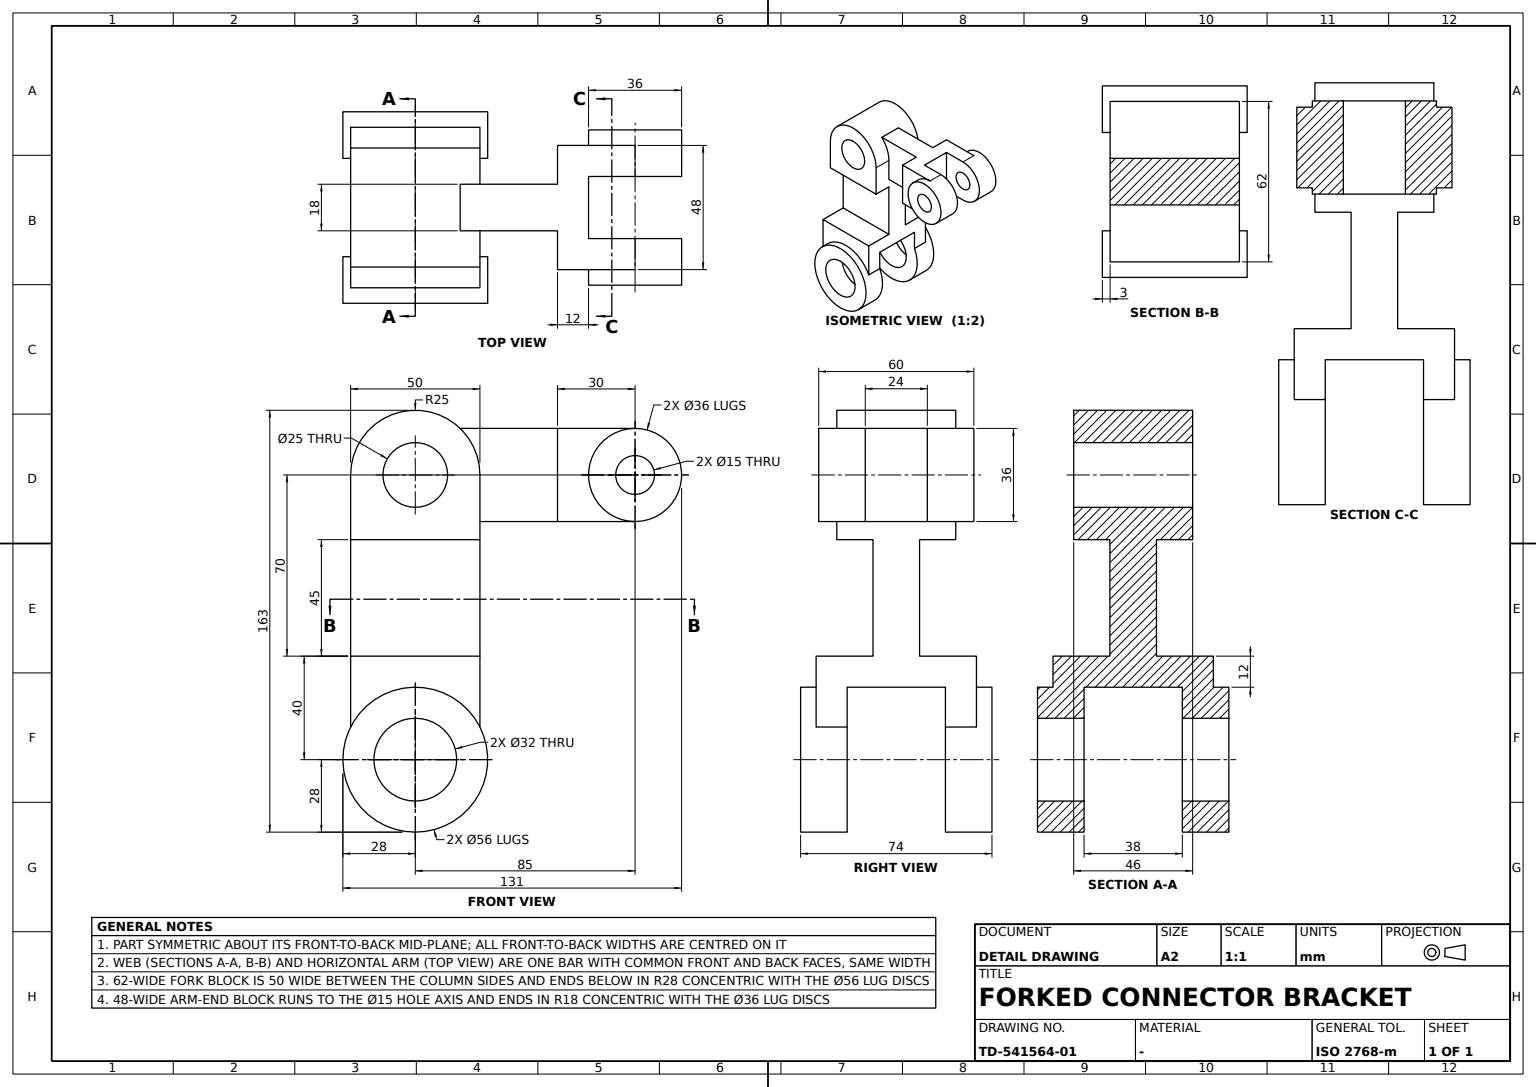
ISO-10303-21;
HEADER;
FILE_DESCRIPTION((''),'2;1');
FILE_NAME('','',(''),(''),'','','');
FILE_SCHEMA(('AUTOMOTIVE_DESIGN'));
ENDSEC;
DATA;
#1=APPLICATION_CONTEXT('');
#2=PRODUCT_CONTEXT('',#1,'mechanical');
#3=PRODUCT('','','',(#2));
#4=PRODUCT_DEFINITION_FORMATION('','',#3);
#5=PRODUCT_DEFINITION_CONTEXT('',#1,'design');
#6=PRODUCT_DEFINITION('','',#4,#5);
#7=PRODUCT_DEFINITION_SHAPE('','',#6);
#8=(LENGTH_UNIT()NAMED_UNIT(*)SI_UNIT(.MILLI.,.METRE.));
#9=(NAMED_UNIT(*)PLANE_ANGLE_UNIT()SI_UNIT($,.RADIAN.));
#10=(NAMED_UNIT(*)SI_UNIT($,.STERADIAN.)SOLID_ANGLE_UNIT());
#11=UNCERTAINTY_MEASURE_WITH_UNIT(LENGTH_MEASURE(0.005),#8,'distance_accuracy_value','');
#12=(GEOMETRIC_REPRESENTATION_CONTEXT(3)GLOBAL_UNCERTAINTY_ASSIGNED_CONTEXT((#11))GLOBAL_UNIT_ASSIGNED_CONTEXT((#8,#9,#10))REPRESENTATION_CONTEXT('',''));
#13=CARTESIAN_POINT('',(-25.,-9.,15.));
#14=VERTEX_POINT('',#13);
#15=CARTESIAN_POINT('',(25.,-9.,15.));
#16=VERTEX_POINT('',#15);
#17=CARTESIAN_POINT('',(0.,-9.,15.));
#18=DIRECTION('',(1.,0.,0.));
#19=VECTOR('',#18,1000.);
#20=LINE('',#17,#19);
#21=EDGE_CURVE('',#14,#16,#20,.T.);
#22=ORIENTED_EDGE('',*,*,#21,.T.);
#23=CARTESIAN_POINT('',(25.,-9.,60.));
#24=VERTEX_POINT('',#23);
#25=CARTESIAN_POINT('',(25.,-9.,0.));
#26=DIRECTION('',(0.,0.,1.));
#27=VECTOR('',#26,1000.);
#28=LINE('',#25,#27);
#29=EDGE_CURVE('',#16,#24,#28,.T.);
#30=ORIENTED_EDGE('',*,*,#29,.T.);
#31=CARTESIAN_POINT('',(-25.,-9.,60.));
#32=VERTEX_POINT('',#31);
#33=CARTESIAN_POINT('',(0.,-9.,60.));
#34=LINE('',#33,#19);
#35=EDGE_CURVE('',#32,#24,#34,.T.);
#36=ORIENTED_EDGE('',*,*,#35,.F.);
#37=CARTESIAN_POINT('',(-25.,-9.,0.));
#38=LINE('',#37,#27);
#39=EDGE_CURVE('',#14,#32,#38,.T.);
#40=ORIENTED_EDGE('',*,*,#39,.F.);
#41=EDGE_LOOP('',(#22,#30,#36,#40));
#42=FACE_BOUND('',#41,.T.);
#43=DIRECTION('',(0.,1.,0.));
#44=AXIS2_PLACEMENT_3D('',#17,#43,#26);
#45=PLANE('',#44);
#46=ADVANCED_FACE('',(#42),#45,.F.);
#47=CARTESIAN_POINT('',(-25.,-23.,85.));
#48=VERTEX_POINT('',#47);
#49=CARTESIAN_POINT('',(25.,-23.,85.));
#50=VERTEX_POINT('',#49);
#51=CARTESIAN_POINT('',(0.,-23.,85.));
#52=AXIS2_PLACEMENT_3D('',#51,#43,#26);
#53=CIRCLE('',#52,25.);
#54=EDGE_CURVE('',#48,#50,#53,.T.);
#55=ORIENTED_EDGE('',*,*,#54,.F.);
#56=CARTESIAN_POINT('',(-25.,-23.,60.));
#57=VERTEX_POINT('',#56);
#58=CARTESIAN_POINT('',(-25.,-23.,0.));
#59=LINE('',#58,#27);
#60=EDGE_CURVE('',#57,#48,#59,.T.);
#61=ORIENTED_EDGE('',*,*,#60,.F.);
#62=CARTESIAN_POINT('',(25.,-23.,60.));
#63=VERTEX_POINT('',#62);
#64=CARTESIAN_POINT('',(0.,-23.,60.));
#65=LINE('',#64,#19);
#66=EDGE_CURVE('',#57,#63,#65,.T.);
#67=ORIENTED_EDGE('',*,*,#66,.T.);
#68=CARTESIAN_POINT('',(25.,-23.,0.));
#69=LINE('',#68,#27);
#70=EDGE_CURVE('',#63,#50,#69,.T.);
#71=ORIENTED_EDGE('',*,*,#70,.T.);
#72=EDGE_LOOP('',(#55,#61,#67,#71));
#73=FACE_BOUND('',#72,.T.);
#74=CARTESIAN_POINT('',(0.,-23.,97.5));
#75=VERTEX_POINT('',#74);
#76=CIRCLE('',#52,12.5);
#77=EDGE_CURVE('',#75,#75,#76,.T.);
#78=ORIENTED_EDGE('',*,*,#77,.T.);
#79=EDGE_LOOP('',(#78));
#80=FACE_BOUND('',#79,.T.);
#81=CARTESIAN_POINT('',(0.,-23.,0.));
#82=DIRECTION('',(-1.,0.,0.));
#83=AXIS2_PLACEMENT_3D('',#81,#43,#82);
#84=PLANE('',#83);
#85=ADVANCED_FACE('',(#73,#80),#84,.F.);
#86=CARTESIAN_POINT('',(85.,-24.,67.));
#87=VERTEX_POINT('',#86);
#88=CARTESIAN_POINT('',(85.,-24.,103.));
#89=VERTEX_POINT('',#88);
#90=CARTESIAN_POINT('',(85.,-24.,85.));
#91=AXIS2_PLACEMENT_3D('',#90,#43,#26);
#92=CIRCLE('',#91,18.);
#93=EDGE_CURVE('',#87,#89,#92,.T.);
#94=ORIENTED_EDGE('',*,*,#93,.T.);
#95=CARTESIAN_POINT('',(55.,-24.,103.));
#96=VERTEX_POINT('',#95);
#97=CARTESIAN_POINT('',(0.,-24.,103.));
#98=LINE('',#97,#19);
#99=EDGE_CURVE('',#96,#89,#98,.T.);
#100=ORIENTED_EDGE('',*,*,#99,.F.);
#101=CARTESIAN_POINT('',(55.,-24.,67.));
#102=VERTEX_POINT('',#101);
#103=CARTESIAN_POINT('',(55.,-24.,85.));
#104=DIRECTION('',(0.,0.,-1.));
#105=VECTOR('',#104,1000.);
#106=LINE('',#103,#105);
#107=EDGE_CURVE('',#96,#102,#106,.T.);
#108=ORIENTED_EDGE('',*,*,#107,.T.);
#109=CARTESIAN_POINT('',(0.,-24.,67.));
#110=LINE('',#109,#19);
#111=EDGE_CURVE('',#102,#87,#110,.T.);
#112=ORIENTED_EDGE('',*,*,#111,.T.);
#113=EDGE_LOOP('',(#94,#100,#108,#112));
#114=FACE_BOUND('',#113,.T.);
#115=AXIS2_PLACEMENT_3D('',#103,#43,#18);
#116=PLANE('',#115);
#117=ADVANCED_FACE('',(#114),#116,.F.);
#118=CARTESIAN_POINT('',(25.,9.,15.));
#119=VERTEX_POINT('',#118);
#120=CARTESIAN_POINT('',(25.,31.,15.));
#121=VERTEX_POINT('',#120);
#122=CARTESIAN_POINT('',(25.,0.,15.));
#123=VECTOR('',#43,1000.);
#124=LINE('',#122,#123);
#125=EDGE_CURVE('',#119,#121,#124,.T.);
#126=ORIENTED_EDGE('',*,*,#125,.T.);
#127=CARTESIAN_POINT('',(-25.,31.,15.));
#128=VERTEX_POINT('',#127);
#129=CARTESIAN_POINT('',(0.,31.,15.));
#130=LINE('',#129,#19);
#131=EDGE_CURVE('',#128,#121,#130,.T.);
#132=ORIENTED_EDGE('',*,*,#131,.F.);
#133=CARTESIAN_POINT('',(-25.,9.,15.));
#134=VERTEX_POINT('',#133);
#135=CARTESIAN_POINT('',(-25.,0.,15.));
#136=LINE('',#135,#123);
#137=EDGE_CURVE('',#134,#128,#136,.T.);
#138=ORIENTED_EDGE('',*,*,#137,.F.);
#139=CARTESIAN_POINT('',(0.,9.,15.));
#140=LINE('',#139,#19);
#141=EDGE_CURVE('',#134,#119,#140,.T.);
#142=ORIENTED_EDGE('',*,*,#141,.T.);
#143=EDGE_LOOP('',(#126,#132,#138,#142));
#144=FACE_BOUND('',#143,.T.);
#145=AXIS2_PLACEMENT_3D('',#139,#104,#43);
#146=PLANE('',#145);
#147=ADVANCED_FACE('',(#144),#146,.F.);
#148=ORIENTED_EDGE('',*,*,#99,.T.);
#149=CARTESIAN_POINT('',(85.,-12.,103.));
#150=VERTEX_POINT('',#149);
#151=CARTESIAN_POINT('',(85.,-21.,103.));
#152=LINE('',#151,#123);
#153=EDGE_CURVE('',#150,#89,#152,.F.);
#154=ORIENTED_EDGE('',*,*,#153,.F.);
#155=CARTESIAN_POINT('',(67.,-12.,103.));
#156=VERTEX_POINT('',#155);
#157=CARTESIAN_POINT('',(0.,-12.,103.));
#158=VECTOR('',#82,1000.);
#159=LINE('',#157,#158);
#160=EDGE_CURVE('',#150,#156,#159,.T.);
#161=ORIENTED_EDGE('',*,*,#160,.T.);
#162=CARTESIAN_POINT('',(67.,12.,103.));
#163=VERTEX_POINT('',#162);
#164=CARTESIAN_POINT('',(67.,0.,103.));
#165=LINE('',#164,#123);
#166=EDGE_CURVE('',#156,#163,#165,.T.);
#167=ORIENTED_EDGE('',*,*,#166,.T.);
#168=CARTESIAN_POINT('',(85.,12.,103.));
#169=VERTEX_POINT('',#168);
#170=CARTESIAN_POINT('',(0.,12.,103.));
#171=LINE('',#170,#158);
#172=EDGE_CURVE('',#169,#163,#171,.T.);
#173=ORIENTED_EDGE('',*,*,#172,.F.);
#174=CARTESIAN_POINT('',(85.,24.,103.));
#175=VERTEX_POINT('',#174);
#176=EDGE_CURVE('',#169,#175,#152,.T.);
#177=ORIENTED_EDGE('',*,*,#176,.T.);
#178=CARTESIAN_POINT('',(55.,24.,103.));
#179=VERTEX_POINT('',#178);
#180=CARTESIAN_POINT('',(0.,24.,103.));
#181=LINE('',#180,#158);
#182=EDGE_CURVE('',#175,#179,#181,.T.);
#183=ORIENTED_EDGE('',*,*,#182,.T.);
#184=CARTESIAN_POINT('',(55.,9.,103.));
#185=VERTEX_POINT('',#184);
#186=CARTESIAN_POINT('',(55.,0.,103.));
#187=DIRECTION('',(0.,-1.,0.));
#188=VECTOR('',#187,1000.);
#189=LINE('',#186,#188);
#190=EDGE_CURVE('',#179,#185,#189,.T.);
#191=ORIENTED_EDGE('',*,*,#190,.T.);
#192=CARTESIAN_POINT('',(17.349352,9.,103.));
#193=VERTEX_POINT('',#192);
#194=CARTESIAN_POINT('',(0.,9.,103.));
#195=LINE('',#194,#158);
#196=EDGE_CURVE('',#185,#193,#195,.T.);
#197=ORIENTED_EDGE('',*,*,#196,.T.);
#198=CARTESIAN_POINT('',(17.349352,-9.,103.));
#199=VERTEX_POINT('',#198);
#200=LINE('',#192,#123);
#201=EDGE_CURVE('',#193,#199,#200,.F.);
#202=ORIENTED_EDGE('',*,*,#201,.T.);
#203=CARTESIAN_POINT('',(55.,-9.,103.));
#204=VERTEX_POINT('',#203);
#205=CARTESIAN_POINT('',(0.,-9.,103.));
#206=LINE('',#205,#19);
#207=EDGE_CURVE('',#199,#204,#206,.T.);
#208=ORIENTED_EDGE('',*,*,#207,.T.);
#209=EDGE_CURVE('',#204,#96,#189,.T.);
#210=ORIENTED_EDGE('',*,*,#209,.T.);
#211=EDGE_LOOP('',(#148,#154,#161,#167,#173,#177,#183,#191,#197,#202,#208,#210));
#212=FACE_BOUND('',#211,.T.);
#213=CARTESIAN_POINT('',(0.,0.,103.));
#214=AXIS2_PLACEMENT_3D('',#213,#104,#18);
#215=PLANE('',#214);
#216=ADVANCED_FACE('',(#212),#215,.F.);
#217=CARTESIAN_POINT('',(85.,12.,67.));
#218=VERTEX_POINT('',#217);
#219=CARTESIAN_POINT('',(85.,24.,67.));
#220=VERTEX_POINT('',#219);
#221=CARTESIAN_POINT('',(85.,-21.,67.));
#222=LINE('',#221,#123);
#223=EDGE_CURVE('',#218,#220,#222,.T.);
#224=ORIENTED_EDGE('',*,*,#223,.F.);
#225=CARTESIAN_POINT('',(67.,12.,67.));
#226=VERTEX_POINT('',#225);
#227=CARTESIAN_POINT('',(0.,12.,67.));
#228=LINE('',#227,#158);
#229=EDGE_CURVE('',#218,#226,#228,.T.);
#230=ORIENTED_EDGE('',*,*,#229,.T.);
#231=CARTESIAN_POINT('',(67.,-12.,67.));
#232=VERTEX_POINT('',#231);
#233=CARTESIAN_POINT('',(67.,0.,67.));
#234=LINE('',#233,#123);
#235=EDGE_CURVE('',#232,#226,#234,.T.);
#236=ORIENTED_EDGE('',*,*,#235,.F.);
#237=CARTESIAN_POINT('',(85.,-12.,67.));
#238=VERTEX_POINT('',#237);
#239=CARTESIAN_POINT('',(0.,-12.,67.));
#240=LINE('',#239,#158);
#241=EDGE_CURVE('',#238,#232,#240,.T.);
#242=ORIENTED_EDGE('',*,*,#241,.F.);
#243=EDGE_CURVE('',#238,#87,#222,.F.);
#244=ORIENTED_EDGE('',*,*,#243,.T.);
#245=ORIENTED_EDGE('',*,*,#111,.F.);
#246=CARTESIAN_POINT('',(55.,-9.,67.));
#247=VERTEX_POINT('',#246);
#248=CARTESIAN_POINT('',(55.,0.,67.));
#249=LINE('',#248,#188);
#250=EDGE_CURVE('',#247,#102,#249,.T.);
#251=ORIENTED_EDGE('',*,*,#250,.F.);
#252=CARTESIAN_POINT('',(25.,-9.,67.));
#253=VERTEX_POINT('',#252);
#254=CARTESIAN_POINT('',(0.,-9.,67.));
#255=LINE('',#254,#19);
#256=EDGE_CURVE('',#253,#247,#255,.T.);
#257=ORIENTED_EDGE('',*,*,#256,.F.);
#258=CARTESIAN_POINT('',(25.,9.,67.));
#259=VERTEX_POINT('',#258);
#260=CARTESIAN_POINT('',(25.,0.,67.));
#261=LINE('',#260,#188);
#262=EDGE_CURVE('',#259,#253,#261,.T.);
#263=ORIENTED_EDGE('',*,*,#262,.F.);
#264=CARTESIAN_POINT('',(55.,9.,67.));
#265=VERTEX_POINT('',#264);
#266=CARTESIAN_POINT('',(0.,9.,67.));
#267=LINE('',#266,#158);
#268=EDGE_CURVE('',#265,#259,#267,.T.);
#269=ORIENTED_EDGE('',*,*,#268,.F.);
#270=CARTESIAN_POINT('',(55.,24.,67.));
#271=VERTEX_POINT('',#270);
#272=EDGE_CURVE('',#271,#265,#249,.T.);
#273=ORIENTED_EDGE('',*,*,#272,.F.);
#274=CARTESIAN_POINT('',(0.,24.,67.));
#275=LINE('',#274,#158);
#276=EDGE_CURVE('',#220,#271,#275,.T.);
#277=ORIENTED_EDGE('',*,*,#276,.F.);
#278=EDGE_LOOP('',(#224,#230,#236,#242,#244,#245,#251,#257,#263,#269,#273,#277));
#279=FACE_BOUND('',#278,.T.);
#280=CARTESIAN_POINT('',(0.,0.,67.));
#281=AXIS2_PLACEMENT_3D('',#280,#104,#18);
#282=PLANE('',#281);
#283=ADVANCED_FACE('',(#279),#282,.T.);
#284=CARTESIAN_POINT('',(0.,19.,-9.));
#285=VERTEX_POINT('',#284);
#286=CARTESIAN_POINT('',(0.,19.,-25.));
#287=AXIS2_PLACEMENT_3D('',#286,#43,#26);
#288=CIRCLE('',#287,16.);
#289=EDGE_CURVE('',#285,#285,#288,.T.);
#290=ORIENTED_EDGE('',*,*,#289,.T.);
#291=EDGE_LOOP('',(#290));
#292=FACE_BOUND('',#291,.T.);
#293=CARTESIAN_POINT('',(-25.,19.,-12.39048));
#294=VERTEX_POINT('',#293);
#295=CARTESIAN_POINT('',(-25.,19.,3.));
#296=VERTEX_POINT('',#295);
#297=CARTESIAN_POINT('',(-25.,19.,0.));
#298=LINE('',#297,#27);
#299=EDGE_CURVE('',#294,#296,#298,.T.);
#300=ORIENTED_EDGE('',*,*,#299,.F.);
#301=CARTESIAN_POINT('',(25.,19.,-12.39048));
#302=VERTEX_POINT('',#301);
#303=CIRCLE('',#287,28.);
#304=EDGE_CURVE('',#294,#302,#303,.F.);
#305=ORIENTED_EDGE('',*,*,#304,.T.);
#306=CARTESIAN_POINT('',(25.,19.,3.));
#307=VERTEX_POINT('',#306);
#308=CARTESIAN_POINT('',(25.,19.,0.));
#309=LINE('',#308,#27);
#310=EDGE_CURVE('',#302,#307,#309,.T.);
#311=ORIENTED_EDGE('',*,*,#310,.T.);
#312=CARTESIAN_POINT('',(0.,19.,3.));
#313=LINE('',#312,#19);
#314=EDGE_CURVE('',#296,#307,#313,.T.);
#315=ORIENTED_EDGE('',*,*,#314,.F.);
#316=EDGE_LOOP('',(#300,#305,#311,#315));
#317=FACE_BOUND('',#316,.T.);
#318=CARTESIAN_POINT('',(0.,19.,-15.));
#319=AXIS2_PLACEMENT_3D('',#318,#43,#26);
#320=PLANE('',#319);
#321=ADVANCED_FACE('',(#292,#317),#320,.F.);
#322=CARTESIAN_POINT('',(0.,-19.,-9.));
#323=VERTEX_POINT('',#322);
#324=CARTESIAN_POINT('',(0.,-19.,-25.));
#325=AXIS2_PLACEMENT_3D('',#324,#43,#26);
#326=CIRCLE('',#325,16.);
#327=EDGE_CURVE('',#323,#323,#326,.T.);
#328=ORIENTED_EDGE('',*,*,#327,.T.);
#329=EDGE_LOOP('',(#328));
#330=FACE_BOUND('',#329,.T.);
#331=CARTESIAN_POINT('',(0.,-37.,-41.));
#332=VERTEX_POINT('',#331);
#333=CARTESIAN_POINT('',(0.,-37.,-25.));
#334=AXIS2_PLACEMENT_3D('',#333,#187,#104);
#335=CIRCLE('',#334,16.);
#336=EDGE_CURVE('',#332,#332,#335,.T.);
#337=ORIENTED_EDGE('',*,*,#336,.T.);
#338=EDGE_LOOP('',(#337));
#339=FACE_BOUND('',#338,.T.);
#340=CARTESIAN_POINT('',(0.,-3.,-25.));
#341=AXIS2_PLACEMENT_3D('',#340,#43,#82);
#342=CYLINDRICAL_SURFACE('',#341,16.);
#343=ADVANCED_FACE('',(#330,#339),#342,.F.);
#344=ORIENTED_EDGE('',*,*,#314,.T.);
#345=CARTESIAN_POINT('',(25.,-19.,3.));
#346=VERTEX_POINT('',#345);
#347=CARTESIAN_POINT('',(25.,0.,3.));
#348=LINE('',#347,#123);
#349=EDGE_CURVE('',#346,#307,#348,.T.);
#350=ORIENTED_EDGE('',*,*,#349,.F.);
#351=CARTESIAN_POINT('',(-25.,-19.,3.));
#352=VERTEX_POINT('',#351);
#353=CARTESIAN_POINT('',(0.,-19.,3.));
#354=LINE('',#353,#19);
#355=EDGE_CURVE('',#352,#346,#354,.T.);
#356=ORIENTED_EDGE('',*,*,#355,.F.);
#357=CARTESIAN_POINT('',(-25.,0.,3.));
#358=LINE('',#357,#123);
#359=EDGE_CURVE('',#352,#296,#358,.T.);
#360=ORIENTED_EDGE('',*,*,#359,.T.);
#361=EDGE_LOOP('',(#344,#350,#356,#360));
#362=FACE_BOUND('',#361,.T.);
#363=AXIS2_PLACEMENT_3D('',#353,#104,#43);
#364=PLANE('',#363);
#365=ADVANCED_FACE('',(#362),#364,.T.);
#366=CARTESIAN_POINT('',(-25.,9.,60.));
#367=VERTEX_POINT('',#366);
#368=CARTESIAN_POINT('',(-25.,9.,0.));
#369=LINE('',#368,#105);
#370=EDGE_CURVE('',#367,#134,#369,.T.);
#371=ORIENTED_EDGE('',*,*,#370,.F.);
#372=CARTESIAN_POINT('',(25.,9.,60.));
#373=VERTEX_POINT('',#372);
#374=CARTESIAN_POINT('',(0.,9.,60.));
#375=LINE('',#374,#19);
#376=EDGE_CURVE('',#367,#373,#375,.T.);
#377=ORIENTED_EDGE('',*,*,#376,.T.);
#378=CARTESIAN_POINT('',(25.,9.,0.));
#379=LINE('',#378,#105);
#380=EDGE_CURVE('',#373,#119,#379,.T.);
#381=ORIENTED_EDGE('',*,*,#380,.T.);
#382=ORIENTED_EDGE('',*,*,#141,.F.);
#383=EDGE_LOOP('',(#371,#377,#381,#382));
#384=FACE_BOUND('',#383,.T.);
#385=AXIS2_PLACEMENT_3D('',#374,#187,#104);
#386=PLANE('',#385);
#387=ADVANCED_FACE('',(#384),#386,.F.);
#388=CARTESIAN_POINT('',(85.,-12.,77.5));
#389=VERTEX_POINT('',#388);
#390=CARTESIAN_POINT('',(85.,-12.,85.));
#391=AXIS2_PLACEMENT_3D('',#390,#187,#104);
#392=CIRCLE('',#391,7.5);
#393=EDGE_CURVE('',#389,#389,#392,.T.);
#394=ORIENTED_EDGE('',*,*,#393,.T.);
#395=EDGE_LOOP('',(#394));
#396=FACE_BOUND('',#395,.T.);
#397=CARTESIAN_POINT('',(67.,-12.,85.));
#398=LINE('',#397,#105);
#399=EDGE_CURVE('',#156,#232,#398,.T.);
#400=ORIENTED_EDGE('',*,*,#399,.F.);
#401=ORIENTED_EDGE('',*,*,#160,.F.);
#402=CIRCLE('',#391,18.);
#403=EDGE_CURVE('',#150,#238,#402,.F.);
#404=ORIENTED_EDGE('',*,*,#403,.T.);
#405=ORIENTED_EDGE('',*,*,#241,.T.);
#406=EDGE_LOOP('',(#400,#401,#404,#405));
#407=FACE_BOUND('',#406,.T.);
#408=AXIS2_PLACEMENT_3D('',#390,#187,#82);
#409=PLANE('',#408);
#410=ADVANCED_FACE('',(#396,#407),#409,.F.);
#411=CARTESIAN_POINT('',(-25.,-19.,-12.39048));
#412=VERTEX_POINT('',#411);
#413=CARTESIAN_POINT('',(-25.,-19.,0.));
#414=LINE('',#413,#27);
#415=EDGE_CURVE('',#412,#352,#414,.T.);
#416=ORIENTED_EDGE('',*,*,#415,.T.);
#417=ORIENTED_EDGE('',*,*,#355,.T.);
#418=CARTESIAN_POINT('',(25.,-19.,-12.39048));
#419=VERTEX_POINT('',#418);
#420=CARTESIAN_POINT('',(25.,-19.,0.));
#421=LINE('',#420,#27);
#422=EDGE_CURVE('',#419,#346,#421,.T.);
#423=ORIENTED_EDGE('',*,*,#422,.F.);
#424=CIRCLE('',#325,28.);
#425=EDGE_CURVE('',#412,#419,#424,.F.);
#426=ORIENTED_EDGE('',*,*,#425,.F.);
#427=EDGE_LOOP('',(#416,#417,#423,#426));
#428=FACE_BOUND('',#427,.T.);
#429=ORIENTED_EDGE('',*,*,#327,.F.);
#430=EDGE_LOOP('',(#429));
#431=FACE_BOUND('',#430,.T.);
#432=CARTESIAN_POINT('',(0.,-19.,-15.));
#433=AXIS2_PLACEMENT_3D('',#432,#43,#26);
#434=PLANE('',#433);
#435=ADVANCED_FACE('',(#428,#431),#434,.T.);
#436=CARTESIAN_POINT('',(85.,-30.,92.5));
#437=VERTEX_POINT('',#436);
#438=CARTESIAN_POINT('',(85.,-30.,85.));
#439=AXIS2_PLACEMENT_3D('',#438,#43,#26);
#440=CIRCLE('',#439,7.5);
#441=EDGE_CURVE('',#437,#437,#440,.T.);
#442=ORIENTED_EDGE('',*,*,#441,.F.);
#443=EDGE_LOOP('',(#442));
#444=FACE_BOUND('',#443,.T.);
#445=ORIENTED_EDGE('',*,*,#393,.F.);
#446=EDGE_LOOP('',(#445));
#447=FACE_BOUND('',#446,.T.);
#448=CARTESIAN_POINT('',(85.,-21.,85.));
#449=AXIS2_PLACEMENT_3D('',#448,#43,#82);
#450=CYLINDRICAL_SURFACE('',#449,7.5);
#451=ADVANCED_FACE('',(#444,#447),#450,.F.);
#452=CARTESIAN_POINT('',(55.,-9.,15.));
#453=LINE('',#452,#105);
#454=EDGE_CURVE('',#204,#247,#453,.T.);
#455=ORIENTED_EDGE('',*,*,#454,.T.);
#456=ORIENTED_EDGE('',*,*,#250,.T.);
#457=ORIENTED_EDGE('',*,*,#107,.F.);
#458=ORIENTED_EDGE('',*,*,#209,.F.);
#459=EDGE_LOOP('',(#455,#456,#457,#458));
#460=FACE_BOUND('',#459,.T.);
#461=CARTESIAN_POINT('',(55.,24.,85.));
#462=AXIS2_PLACEMENT_3D('',#461,#18,#187);
#463=PLANE('',#462);
#464=ADVANCED_FACE('',(#460),#463,.F.);
#465=ORIENTED_EDGE('',*,*,#289,.F.);
#466=EDGE_LOOP('',(#465));
#467=FACE_BOUND('',#466,.T.);
#468=CARTESIAN_POINT('',(0.,37.,-41.));
#469=VERTEX_POINT('',#468);
#470=CARTESIAN_POINT('',(0.,37.,-25.));
#471=AXIS2_PLACEMENT_3D('',#470,#187,#104);
#472=CIRCLE('',#471,16.);
#473=EDGE_CURVE('',#469,#469,#472,.T.);
#474=ORIENTED_EDGE('',*,*,#473,.F.);
#475=EDGE_LOOP('',(#474));
#476=FACE_BOUND('',#475,.T.);
#477=ADVANCED_FACE('',(#467,#476),#342,.F.);
#478=CARTESIAN_POINT('',(0.,37.,-53.));
#479=VERTEX_POINT('',#478);
#480=CIRCLE('',#471,28.);
#481=EDGE_CURVE('',#479,#479,#480,.T.);
#482=ORIENTED_EDGE('',*,*,#481,.F.);
#483=EDGE_LOOP('',(#482));
#484=FACE_BOUND('',#483,.T.);
#485=ORIENTED_EDGE('',*,*,#473,.T.);
#486=EDGE_LOOP('',(#485));
#487=FACE_BOUND('',#486,.T.);
#488=CARTESIAN_POINT('',(0.,37.,0.));
#489=AXIS2_PLACEMENT_3D('',#488,#187,#18);
#490=PLANE('',#489);
#491=ADVANCED_FACE('',(#484,#487),#490,.F.);
#492=CARTESIAN_POINT('',(-25.,-31.,15.));
#493=VERTEX_POINT('',#492);
#494=EDGE_CURVE('',#493,#14,#136,.T.);
#495=ORIENTED_EDGE('',*,*,#494,.F.);
#496=CARTESIAN_POINT('',(25.,-31.,15.));
#497=VERTEX_POINT('',#496);
#498=CARTESIAN_POINT('',(0.,-31.,15.));
#499=LINE('',#498,#19);
#500=EDGE_CURVE('',#493,#497,#499,.T.);
#501=ORIENTED_EDGE('',*,*,#500,.T.);
#502=EDGE_CURVE('',#497,#16,#124,.T.);
#503=ORIENTED_EDGE('',*,*,#502,.T.);
#504=ORIENTED_EDGE('',*,*,#21,.F.);
#505=EDGE_LOOP('',(#495,#501,#503,#504));
#506=FACE_BOUND('',#505,.T.);
#507=ADVANCED_FACE('',(#506),#146,.F.);
#508=ORIENTED_EDGE('',*,*,#454,.F.);
#509=ORIENTED_EDGE('',*,*,#207,.F.);
#510=CARTESIAN_POINT('',(25.,-9.,85.));
#511=VERTEX_POINT('',#510);
#512=CARTESIAN_POINT('',(0.,-9.,85.));
#513=AXIS2_PLACEMENT_3D('',#512,#43,#26);
#514=CIRCLE('',#513,25.);
#515=EDGE_CURVE('',#199,#511,#514,.T.);
#516=ORIENTED_EDGE('',*,*,#515,.T.);
#517=LINE('',#15,#105);
#518=EDGE_CURVE('',#511,#253,#517,.T.);
#519=ORIENTED_EDGE('',*,*,#518,.T.);
#520=ORIENTED_EDGE('',*,*,#256,.T.);
#521=EDGE_LOOP('',(#508,#509,#516,#519,#520));
#522=FACE_BOUND('',#521,.T.);
#523=ADVANCED_FACE('',(#522),#45,.F.);
#524=LINE('',#461,#105);
#525=EDGE_CURVE('',#179,#271,#524,.T.);
#526=ORIENTED_EDGE('',*,*,#525,.T.);
#527=ORIENTED_EDGE('',*,*,#272,.T.);
#528=CARTESIAN_POINT('',(55.,9.,85.));
#529=LINE('',#528,#105);
#530=EDGE_CURVE('',#185,#265,#529,.T.);
#531=ORIENTED_EDGE('',*,*,#530,.F.);
#532=ORIENTED_EDGE('',*,*,#190,.F.);
#533=EDGE_LOOP('',(#526,#527,#531,#532));
#534=FACE_BOUND('',#533,.T.);
#535=ADVANCED_FACE('',(#534),#463,.F.);
#536=CARTESIAN_POINT('',(67.,12.,85.));
#537=LINE('',#536,#105);
#538=EDGE_CURVE('',#163,#226,#537,.T.);
#539=ORIENTED_EDGE('',*,*,#538,.F.);
#540=ORIENTED_EDGE('',*,*,#166,.F.);
#541=ORIENTED_EDGE('',*,*,#399,.T.);
#542=ORIENTED_EDGE('',*,*,#235,.T.);
#543=EDGE_LOOP('',(#539,#540,#541,#542));
#544=FACE_BOUND('',#543,.T.);
#545=AXIS2_PLACEMENT_3D('',#397,#82,#43);
#546=PLANE('',#545);
#547=ADVANCED_FACE('',(#544),#546,.F.);
#548=ORIENTED_EDGE('',*,*,#403,.F.);
#549=ORIENTED_EDGE('',*,*,#153,.T.);
#550=ORIENTED_EDGE('',*,*,#93,.F.);
#551=ORIENTED_EDGE('',*,*,#243,.F.);
#552=EDGE_LOOP('',(#548,#549,#550,#551));
#553=FACE_BOUND('',#552,.T.);
#554=CARTESIAN_POINT('',(85.,-30.,103.));
#555=VERTEX_POINT('',#554);
#556=CIRCLE('',#439,18.);
#557=EDGE_CURVE('',#555,#555,#556,.T.);
#558=ORIENTED_EDGE('',*,*,#557,.T.);
#559=EDGE_LOOP('',(#558));
#560=FACE_BOUND('',#559,.T.);
#561=CYLINDRICAL_SURFACE('',#449,18.);
#562=ADVANCED_FACE('',(#553,#560),#561,.T.);
#563=CARTESIAN_POINT('',(92.5,12.,85.));
#564=VERTEX_POINT('',#563);
#565=CARTESIAN_POINT('',(85.,12.,85.));
#566=AXIS2_PLACEMENT_3D('',#565,#187,#18);
#567=CIRCLE('',#566,7.5);
#568=EDGE_CURVE('',#564,#564,#567,.T.);
#569=ORIENTED_EDGE('',*,*,#568,.T.);
#570=EDGE_LOOP('',(#569));
#571=FACE_BOUND('',#570,.T.);
#572=CARTESIAN_POINT('',(85.,30.,92.5));
#573=VERTEX_POINT('',#572);
#574=CARTESIAN_POINT('',(85.,30.,85.));
#575=AXIS2_PLACEMENT_3D('',#574,#43,#26);
#576=CIRCLE('',#575,7.5);
#577=EDGE_CURVE('',#573,#573,#576,.T.);
#578=ORIENTED_EDGE('',*,*,#577,.T.);
#579=EDGE_LOOP('',(#578));
#580=FACE_BOUND('',#579,.T.);
#581=ADVANCED_FACE('',(#571,#580),#450,.F.);
#582=CARTESIAN_POINT('',(25.,0.,60.));
#583=LINE('',#582,#123);
#584=EDGE_CURVE('',#63,#24,#583,.T.);
#585=ORIENTED_EDGE('',*,*,#584,.F.);
#586=ORIENTED_EDGE('',*,*,#66,.F.);
#587=CARTESIAN_POINT('',(-25.,0.,60.));
#588=LINE('',#587,#123);
#589=EDGE_CURVE('',#57,#32,#588,.T.);
#590=ORIENTED_EDGE('',*,*,#589,.T.);
#591=ORIENTED_EDGE('',*,*,#35,.T.);
#592=EDGE_LOOP('',(#585,#586,#590,#591));
#593=FACE_BOUND('',#592,.T.);
#594=AXIS2_PLACEMENT_3D('',#33,#104,#43);
#595=PLANE('',#594);
#596=ADVANCED_FACE('',(#593),#595,.T.);
#597=CARTESIAN_POINT('',(25.,9.,85.));
#598=VERTEX_POINT('',#597);
#599=CARTESIAN_POINT('',(0.,9.,85.));
#600=AXIS2_PLACEMENT_3D('',#599,#187,#104);
#601=CIRCLE('',#600,25.);
#602=EDGE_CURVE('',#598,#193,#601,.T.);
#603=ORIENTED_EDGE('',*,*,#602,.T.);
#604=ORIENTED_EDGE('',*,*,#196,.F.);
#605=ORIENTED_EDGE('',*,*,#530,.T.);
#606=ORIENTED_EDGE('',*,*,#268,.T.);
#607=EDGE_CURVE('',#598,#259,#379,.T.);
#608=ORIENTED_EDGE('',*,*,#607,.F.);
#609=EDGE_LOOP('',(#603,#604,#605,#606,#608));
#610=FACE_BOUND('',#609,.T.);
#611=ADVANCED_FACE('',(#610),#386,.F.);
#612=CARTESIAN_POINT('',(25.,31.,-12.39048));
#613=VERTEX_POINT('',#612);
#614=CARTESIAN_POINT('',(25.,31.,0.));
#615=LINE('',#614,#105);
#616=EDGE_CURVE('',#121,#613,#615,.T.);
#617=ORIENTED_EDGE('',*,*,#616,.F.);
#618=ORIENTED_EDGE('',*,*,#125,.F.);
#619=ORIENTED_EDGE('',*,*,#380,.F.);
#620=CARTESIAN_POINT('',(25.,23.,60.));
#621=VERTEX_POINT('',#620);
#622=EDGE_CURVE('',#373,#621,#583,.T.);
#623=ORIENTED_EDGE('',*,*,#622,.T.);
#624=CARTESIAN_POINT('',(25.,23.,85.));
#625=VERTEX_POINT('',#624);
#626=CARTESIAN_POINT('',(25.,23.,0.));
#627=LINE('',#626,#27);
#628=EDGE_CURVE('',#621,#625,#627,.T.);
#629=ORIENTED_EDGE('',*,*,#628,.T.);
#630=CARTESIAN_POINT('',(25.,0.,85.));
#631=LINE('',#630,#123);
#632=EDGE_CURVE('',#598,#625,#631,.T.);
#633=ORIENTED_EDGE('',*,*,#632,.F.);
#634=ORIENTED_EDGE('',*,*,#607,.T.);
#635=ORIENTED_EDGE('',*,*,#262,.T.);
#636=ORIENTED_EDGE('',*,*,#518,.F.);
#637=EDGE_CURVE('',#50,#511,#631,.T.);
#638=ORIENTED_EDGE('',*,*,#637,.F.);
#639=ORIENTED_EDGE('',*,*,#70,.F.);
#640=ORIENTED_EDGE('',*,*,#584,.T.);
#641=ORIENTED_EDGE('',*,*,#29,.F.);
#642=ORIENTED_EDGE('',*,*,#502,.F.);
#643=CARTESIAN_POINT('',(25.,-31.,-12.39048));
#644=VERTEX_POINT('',#643);
#645=CARTESIAN_POINT('',(25.,-31.,0.));
#646=LINE('',#645,#27);
#647=EDGE_CURVE('',#644,#497,#646,.T.);
#648=ORIENTED_EDGE('',*,*,#647,.F.);
#649=LINE('',#643,#188);
#650=EDGE_CURVE('',#644,#419,#649,.F.);
#651=ORIENTED_EDGE('',*,*,#650,.T.);
#652=ORIENTED_EDGE('',*,*,#422,.T.);
#653=ORIENTED_EDGE('',*,*,#349,.T.);
#654=ORIENTED_EDGE('',*,*,#310,.F.);
#655=LINE('',#612,#188);
#656=EDGE_CURVE('',#613,#302,#655,.T.);
#657=ORIENTED_EDGE('',*,*,#656,.F.);
#658=EDGE_LOOP('',(#617,#618,#619,#623,#629,#633,#634,#635,#636,#638,#639,#640,#641,#642,#648,#651,#652,#653,#654,#657));
#659=FACE_BOUND('',#658,.T.);
#660=CARTESIAN_POINT('',(25.,0.,0.));
#661=AXIS2_PLACEMENT_3D('',#660,#18,#43);
#662=PLANE('',#661);
#663=ADVANCED_FACE('',(#659),#662,.T.);
#664=ORIENTED_EDGE('',*,*,#336,.F.);
#665=EDGE_LOOP('',(#664));
#666=FACE_BOUND('',#665,.T.);
#667=CARTESIAN_POINT('',(0.,-37.,-53.));
#668=VERTEX_POINT('',#667);
#669=CIRCLE('',#334,28.);
#670=EDGE_CURVE('',#668,#668,#669,.T.);
#671=ORIENTED_EDGE('',*,*,#670,.T.);
#672=EDGE_LOOP('',(#671));
#673=FACE_BOUND('',#672,.T.);
#674=CARTESIAN_POINT('',(0.,-37.,0.));
#675=AXIS2_PLACEMENT_3D('',#674,#187,#18);
#676=PLANE('',#675);
#677=ADVANCED_FACE('',(#666,#673),#676,.T.);
#678=CARTESIAN_POINT('',(85.,24.,85.));
#679=AXIS2_PLACEMENT_3D('',#678,#187,#104);
#680=CIRCLE('',#679,18.);
#681=EDGE_CURVE('',#175,#220,#680,.T.);
#682=ORIENTED_EDGE('',*,*,#681,.T.);
#683=ORIENTED_EDGE('',*,*,#276,.T.);
#684=ORIENTED_EDGE('',*,*,#525,.F.);
#685=ORIENTED_EDGE('',*,*,#182,.F.);
#686=EDGE_LOOP('',(#682,#683,#684,#685));
#687=FACE_BOUND('',#686,.T.);
#688=AXIS2_PLACEMENT_3D('',#678,#187,#82);
#689=PLANE('',#688);
#690=ADVANCED_FACE('',(#687),#689,.F.);
#691=CARTESIAN_POINT('',(-25.,-31.,-12.39048));
#692=VERTEX_POINT('',#691);
#693=CARTESIAN_POINT('',(0.,-31.,-25.));
#694=AXIS2_PLACEMENT_3D('',#693,#43,#26);
#695=CIRCLE('',#694,28.);
#696=EDGE_CURVE('',#692,#644,#695,.T.);
#697=ORIENTED_EDGE('',*,*,#696,.F.);
#698=LINE('',#691,#188);
#699=EDGE_CURVE('',#692,#412,#698,.F.);
#700=ORIENTED_EDGE('',*,*,#699,.T.);
#701=ORIENTED_EDGE('',*,*,#425,.T.);
#702=ORIENTED_EDGE('',*,*,#650,.F.);
#703=EDGE_LOOP('',(#697,#700,#701,#702));
#704=FACE_BOUND('',#703,.T.);
#705=ORIENTED_EDGE('',*,*,#670,.F.);
#706=EDGE_LOOP('',(#705));
#707=FACE_BOUND('',#706,.T.);
#708=CARTESIAN_POINT('',(0.,28.,-25.));
#709=AXIS2_PLACEMENT_3D('',#708,#187,#18);
#710=CYLINDRICAL_SURFACE('',#709,28.);
#711=ADVANCED_FACE('',(#704,#707),#710,.T.);
#712=CARTESIAN_POINT('',(85.,30.,103.));
#713=VERTEX_POINT('',#712);
#714=CIRCLE('',#575,18.);
#715=EDGE_CURVE('',#713,#713,#714,.T.);
#716=ORIENTED_EDGE('',*,*,#715,.T.);
#717=EDGE_LOOP('',(#716));
#718=FACE_BOUND('',#717,.T.);
#719=ORIENTED_EDGE('',*,*,#577,.F.);
#720=EDGE_LOOP('',(#719));
#721=FACE_BOUND('',#720,.T.);
#722=CARTESIAN_POINT('',(0.,30.,0.));
#723=AXIS2_PLACEMENT_3D('',#722,#43,#82);
#724=PLANE('',#723);
#725=ADVANCED_FACE('',(#718,#721),#724,.T.);
#726=CARTESIAN_POINT('',(-25.,23.,85.));
#727=VERTEX_POINT('',#726);
#728=CARTESIAN_POINT('',(0.,23.,85.));
#729=AXIS2_PLACEMENT_3D('',#728,#43,#26);
#730=CIRCLE('',#729,25.);
#731=EDGE_CURVE('',#727,#625,#730,.T.);
#732=ORIENTED_EDGE('',*,*,#731,.T.);
#733=ORIENTED_EDGE('',*,*,#628,.F.);
#734=CARTESIAN_POINT('',(-25.,23.,60.));
#735=VERTEX_POINT('',#734);
#736=CARTESIAN_POINT('',(0.,23.,60.));
#737=LINE('',#736,#19);
#738=EDGE_CURVE('',#735,#621,#737,.T.);
#739=ORIENTED_EDGE('',*,*,#738,.F.);
#740=CARTESIAN_POINT('',(-25.,23.,0.));
#741=LINE('',#740,#27);
#742=EDGE_CURVE('',#735,#727,#741,.T.);
#743=ORIENTED_EDGE('',*,*,#742,.T.);
#744=EDGE_LOOP('',(#732,#733,#739,#743));
#745=FACE_BOUND('',#744,.T.);
#746=CARTESIAN_POINT('',(0.,23.,97.5));
#747=VERTEX_POINT('',#746);
#748=CIRCLE('',#729,12.5);
#749=EDGE_CURVE('',#747,#747,#748,.T.);
#750=ORIENTED_EDGE('',*,*,#749,.F.);
#751=EDGE_LOOP('',(#750));
#752=FACE_BOUND('',#751,.T.);
#753=CARTESIAN_POINT('',(0.,23.,0.));
#754=AXIS2_PLACEMENT_3D('',#753,#43,#82);
#755=PLANE('',#754);
#756=ADVANCED_FACE('',(#745,#752),#755,.T.);
#757=ORIENTED_EDGE('',*,*,#715,.F.);
#758=EDGE_LOOP('',(#757));
#759=FACE_BOUND('',#758,.T.);
#760=ORIENTED_EDGE('',*,*,#681,.F.);
#761=ORIENTED_EDGE('',*,*,#176,.F.);
#762=CIRCLE('',#566,18.);
#763=EDGE_CURVE('',#169,#218,#762,.F.);
#764=ORIENTED_EDGE('',*,*,#763,.T.);
#765=ORIENTED_EDGE('',*,*,#223,.T.);
#766=EDGE_LOOP('',(#760,#761,#764,#765));
#767=FACE_BOUND('',#766,.T.);
#768=ADVANCED_FACE('',(#759,#767),#561,.T.);
#769=ORIENTED_EDGE('',*,*,#500,.F.);
#770=CARTESIAN_POINT('',(-25.,-31.,0.));
#771=LINE('',#770,#27);
#772=EDGE_CURVE('',#692,#493,#771,.T.);
#773=ORIENTED_EDGE('',*,*,#772,.F.);
#774=ORIENTED_EDGE('',*,*,#696,.T.);
#775=ORIENTED_EDGE('',*,*,#647,.T.);
#776=EDGE_LOOP('',(#769,#773,#774,#775));
#777=FACE_BOUND('',#776,.T.);
#778=CARTESIAN_POINT('',(0.,-31.,-15.));
#779=AXIS2_PLACEMENT_3D('',#778,#43,#26);
#780=PLANE('',#779);
#781=ADVANCED_FACE('',(#777),#780,.F.);
#782=ORIENTED_EDGE('',*,*,#568,.F.);
#783=EDGE_LOOP('',(#782));
#784=FACE_BOUND('',#783,.T.);
#785=ORIENTED_EDGE('',*,*,#172,.T.);
#786=ORIENTED_EDGE('',*,*,#538,.T.);
#787=ORIENTED_EDGE('',*,*,#229,.F.);
#788=ORIENTED_EDGE('',*,*,#763,.F.);
#789=EDGE_LOOP('',(#785,#786,#787,#788));
#790=FACE_BOUND('',#789,.T.);
#791=AXIS2_PLACEMENT_3D('',#565,#187,#82);
#792=PLANE('',#791);
#793=ADVANCED_FACE('',(#784,#790),#792,.T.);
#794=ORIENTED_EDGE('',*,*,#481,.T.);
#795=EDGE_LOOP('',(#794));
#796=FACE_BOUND('',#795,.T.);
#797=ORIENTED_EDGE('',*,*,#656,.T.);
#798=ORIENTED_EDGE('',*,*,#304,.F.);
#799=CARTESIAN_POINT('',(-25.,31.,-12.39048));
#800=VERTEX_POINT('',#799);
#801=LINE('',#799,#188);
#802=EDGE_CURVE('',#800,#294,#801,.T.);
#803=ORIENTED_EDGE('',*,*,#802,.F.);
#804=CARTESIAN_POINT('',(0.,31.,-25.));
#805=AXIS2_PLACEMENT_3D('',#804,#187,#104);
#806=CIRCLE('',#805,28.);
#807=EDGE_CURVE('',#613,#800,#806,.T.);
#808=ORIENTED_EDGE('',*,*,#807,.F.);
#809=EDGE_LOOP('',(#797,#798,#803,#808));
#810=FACE_BOUND('',#809,.T.);
#811=ADVANCED_FACE('',(#796,#810),#710,.T.);
#812=ORIENTED_EDGE('',*,*,#54,.T.);
#813=ORIENTED_EDGE('',*,*,#637,.T.);
#814=ORIENTED_EDGE('',*,*,#515,.F.);
#815=ORIENTED_EDGE('',*,*,#201,.F.);
#816=ORIENTED_EDGE('',*,*,#602,.F.);
#817=ORIENTED_EDGE('',*,*,#632,.T.);
#818=ORIENTED_EDGE('',*,*,#731,.F.);
#819=CARTESIAN_POINT('',(-25.,0.,85.));
#820=LINE('',#819,#123);
#821=EDGE_CURVE('',#48,#727,#820,.T.);
#822=ORIENTED_EDGE('',*,*,#821,.F.);
#823=EDGE_LOOP('',(#812,#813,#814,#815,#816,#817,#818,#822));
#824=FACE_BOUND('',#823,.T.);
#825=CARTESIAN_POINT('',(0.,0.,85.));
#826=AXIS2_PLACEMENT_3D('',#825,#43,#82);
#827=CYLINDRICAL_SURFACE('',#826,25.);
#828=ADVANCED_FACE('',(#824),#827,.T.);
#829=ORIENTED_EDGE('',*,*,#622,.F.);
#830=ORIENTED_EDGE('',*,*,#376,.F.);
#831=EDGE_CURVE('',#367,#735,#588,.T.);
#832=ORIENTED_EDGE('',*,*,#831,.T.);
#833=ORIENTED_EDGE('',*,*,#738,.T.);
#834=EDGE_LOOP('',(#829,#830,#832,#833));
#835=FACE_BOUND('',#834,.T.);
#836=ADVANCED_FACE('',(#835),#595,.T.);
#837=CARTESIAN_POINT('',(-25.,31.,0.));
#838=LINE('',#837,#105);
#839=EDGE_CURVE('',#128,#800,#838,.T.);
#840=ORIENTED_EDGE('',*,*,#839,.F.);
#841=ORIENTED_EDGE('',*,*,#131,.T.);
#842=ORIENTED_EDGE('',*,*,#616,.T.);
#843=ORIENTED_EDGE('',*,*,#807,.T.);
#844=EDGE_LOOP('',(#840,#841,#842,#843));
#845=FACE_BOUND('',#844,.T.);
#846=AXIS2_PLACEMENT_3D('',#129,#187,#104);
#847=PLANE('',#846);
#848=ADVANCED_FACE('',(#845),#847,.F.);
#849=ORIENTED_EDGE('',*,*,#749,.T.);
#850=EDGE_LOOP('',(#849));
#851=FACE_BOUND('',#850,.T.);
#852=ORIENTED_EDGE('',*,*,#77,.F.);
#853=EDGE_LOOP('',(#852));
#854=FACE_BOUND('',#853,.T.);
#855=CYLINDRICAL_SURFACE('',#826,12.5);
#856=ADVANCED_FACE('',(#851,#854),#855,.F.);
#857=ORIENTED_EDGE('',*,*,#494,.T.);
#858=ORIENTED_EDGE('',*,*,#39,.T.);
#859=ORIENTED_EDGE('',*,*,#589,.F.);
#860=ORIENTED_EDGE('',*,*,#60,.T.);
#861=ORIENTED_EDGE('',*,*,#821,.T.);
#862=ORIENTED_EDGE('',*,*,#742,.F.);
#863=ORIENTED_EDGE('',*,*,#831,.F.);
#864=ORIENTED_EDGE('',*,*,#370,.T.);
#865=ORIENTED_EDGE('',*,*,#137,.T.);
#866=ORIENTED_EDGE('',*,*,#839,.T.);
#867=ORIENTED_EDGE('',*,*,#802,.T.);
#868=ORIENTED_EDGE('',*,*,#299,.T.);
#869=ORIENTED_EDGE('',*,*,#359,.F.);
#870=ORIENTED_EDGE('',*,*,#415,.F.);
#871=ORIENTED_EDGE('',*,*,#699,.F.);
#872=ORIENTED_EDGE('',*,*,#772,.T.);
#873=EDGE_LOOP('',(#857,#858,#859,#860,#861,#862,#863,#864,#865,#866,#867,#868,#869,#870,#871,#872));
#874=FACE_BOUND('',#873,.T.);
#875=CARTESIAN_POINT('',(-25.,0.,0.));
#876=AXIS2_PLACEMENT_3D('',#875,#18,#43);
#877=PLANE('',#876);
#878=ADVANCED_FACE('',(#874),#877,.F.);
#879=ORIENTED_EDGE('',*,*,#441,.T.);
#880=EDGE_LOOP('',(#879));
#881=FACE_BOUND('',#880,.T.);
#882=ORIENTED_EDGE('',*,*,#557,.F.);
#883=EDGE_LOOP('',(#882));
#884=FACE_BOUND('',#883,.T.);
#885=CARTESIAN_POINT('',(0.,-30.,0.));
#886=AXIS2_PLACEMENT_3D('',#885,#43,#82);
#887=PLANE('',#886);
#888=ADVANCED_FACE('',(#881,#884),#887,.F.);
#889=CLOSED_SHELL('',(#46,#85,#117,#147,#216,#283,#321,#343,#365,#387,#410,#435,#451,#464,#477,#491,#507,#523,#535,#547,#562,#581,#596,#611,#663,#677,#690,#711,#725,#756,#768,#781,#793,#811,#828,#836,#848,#856,#878,#888));
#890=MANIFOLD_SOLID_BREP('',#889);
#891=ADVANCED_BREP_SHAPE_REPRESENTATION('',(#890),#12);
#892=SHAPE_DEFINITION_REPRESENTATION(#7,#891);
ENDSEC;
END-ISO-10303-21;
